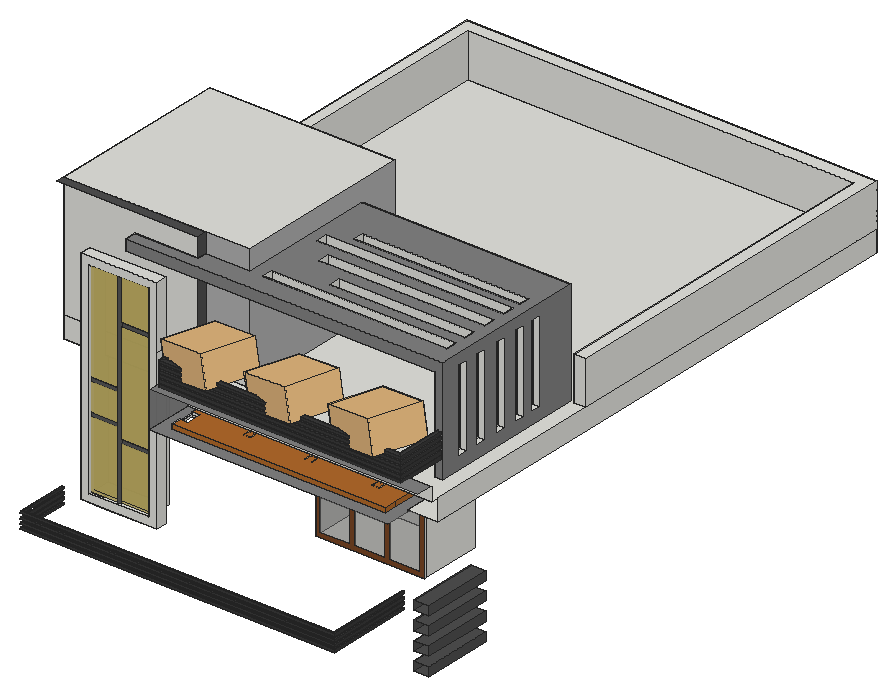
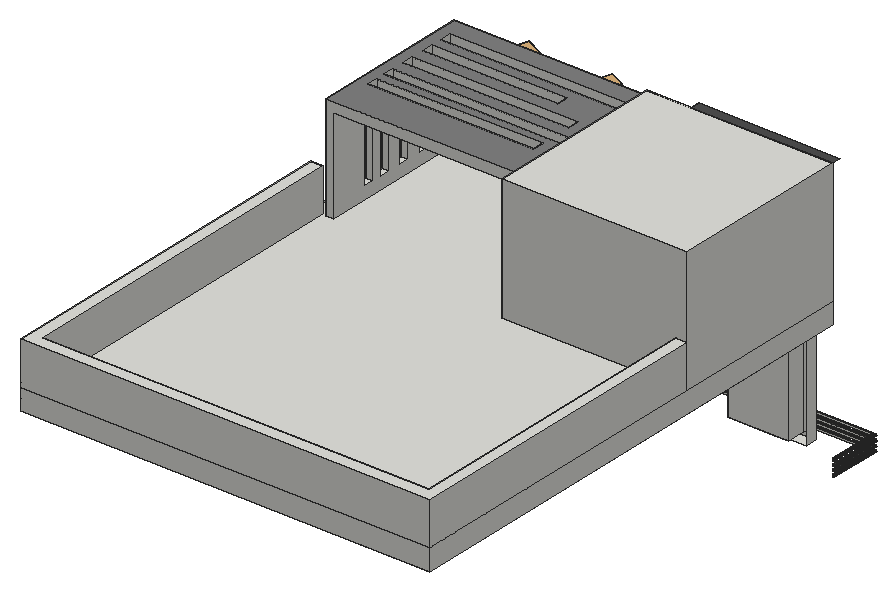
# SketchUp Ruby script. Lengths in inches.
U = 1.inch
M = Sketchup.active_model
def pt(a) = Geom::Point3d.new(a.map { |v| v * U })
def face(e, loops, mat)
  f = e.add_face(loops[0].map { |a| pt(a) })
  loops[1..].each { |l| e.add_face(l.map { |a| pt(a) }).erase! }
  f.material = f.back_material = mat if mat
  f
end
# faces: each face lists its corners as indices into pts; further lists are holes
def faces(e, pts, list, mat = nil) = list.each { |f| face(e, (f[0].is_a?(Array) ? f : [f]).map { |l| l.map { |i| pts[i] } }, mat) }
# xy, xz, yz: faces in a plane at the given z, y or x. An outline is a flat list of corners, or four numbers for a rectangle; further outlines are holes
def ring(l) = l.size == 4 ? [[l[0], l[1]], [l[2], l[1]], [l[2], l[3]], [l[0], l[3]]] : l.each_slice(2).to_a
def flat(e, list, mat, &to3) = list.each { |f| face(e, (f[0].is_a?(Array) ? f : [f]).map { |l| ring(l).map { |u, v| to3.(u, v) } }, mat) }
def xy(e, z, list, mat = nil) = flat(e, list, mat) { |x, y| [x, y, z] }
def xz(e, y, list, mat = nil) = flat(e, list, mat) { |x, z| [x, y, z] }
def yz(e, x, list, mat = nil) = flat(e, list, mat) { |y, z| [x, y, z] }
def lines(e, pts, list) = list.each { |a, b| e.add_line(pt(pts[a]), pt(pts[b])) }
# prism: a flat outline (further loops are holes) pulled along v
def prism(e, loops, v, mat = nil)
  f = face(e, loops, mat); d = Geom::Vector3d.new(v.map { |x| x * U })
  f.pushpull(f.normal.samedirection?(d) ? d.length : -d.length)
end
def box(e, o, s, mat = nil) = prism(e, [[o, [o[0] + s[0], o[1], o[2]], [o[0] + s[0], o[1] + s[1], o[2]], [o[0], o[1] + s[1], o[2]]]], [0, 0, s[2]], mat)
def at(x, y, z, deg = 0) = Geom::Transformation.translation(pt([x, y, z])) * Geom::Transformation.rotation(ORIGIN, Z_AXIS, deg.degrees)
def axes(o, x, y, z) = Geom::Transformation.new([*x, 0, *y, 0, *z, 0, *pt(o).to_a, 1])
def part(name) = M.definitions.add(name)
# library, detail: a bought-in or finely detailed component or shape, given as its bounding box
def library(name, o, s) = part(name).tap { |d| box(d.entities, o, s) }
def detail(e, o, s) = box(e.add_group.entities, o, s)
def put(e, d, t, mat = nil) = e.add_instance(d, t).tap { |i| i.material = mat if mat }
def group(e, t, mat = nil) = e.add_group.tap { |g| g.transformation = t; g.material = mat if mat }.entities
root = M.entities
M.materials.add("Generic").color = [129, 129, 129]
M.materials["Generic"].alpha = 0.97
M.materials.add("Generic\#1").color = [79, 79, 79]
M.materials.add("Generic\#4").color = [176, 176, 176]
M.materials.add("Generic\#6").color = [129, 129, 129]
M.materials.add("Material__1").color = [190, 136, 85]
M.materials.add("Material__2").color = [51, 42, 44]
M.materials.add("Material__3").color = [119, 136, 107]
M.materials.add("[Color M06]").color = [86, 86, 86]
M.materials.add("[Color M07]").color = [196, 178, 100]
M.materials["[Color M07]"].alpha = 0.86
M.materials.add("[Color M07]1").color = [58, 58, 58]
M.materials.add("[Translucent Glass Gray]").color = [128, 128, 128]
M.materials["[Translucent Glass Gray]"].alpha = 0.28
M.materials.add("[Wood Bamboo]").color = [177, 105, 43]
M.materials.add("[Wood Veneer 01]").color = [120, 70, 37]
c1 = library("Tlon Light 450 Ceiling 152 006",[-8.86,-8.86,-3.78],[17.72,17.72,3.56])
c2 = library("\#2",[-119.83,-119.83,113.8],[239.66,239.66,17.4])
c3 = library("\#4",[-204.92,-212.35,-236.71],[424.28,257.5,472.53])
c4 = part("\#3")
put(c4.entities,c3,axes([-0.37,309.72,0],[1.36765,0,0],[0,1.36765,0],[0,0,1.36765]),"Material__3")
c5 = library("\#1",[-174.07,-174.07,0],[348.14,348.14,140])
c6 = part("9")
put(c6.entities,c2,at(-19.94,-24.66,0),"Material__2")
put(c6.entities,c4,axes([17.67,-32.6,40.29],[0.29694,0.9549,0],[-0.21403,0.06656,0.97456],[0.9306,-0.28939,0.22414]))
put(c6.entities,c5,at(-19.94,-24.66,0),"Material__1")
xy(root,181.49,[[80.31,70.4,80.31,115.77,82.18,115.77,82.18,72.28,354.41,72.28,354.41,146.83,356.29,146.83,356.29,70.4]])
xy(root,181.63,[[415.03,84.21,427.87,146.83]],"Generic\#1")
xy(root,183.35,[[80.32,70.42,356.27,70.42,356.27,146.83,354.4,146.83,354.4,72.29,82.2,72.29,82.2,115.77,80.32,115.77]],"[Color M07]1")
xy(root,185.61,[[80.31,70.4,80.31,115.77,82.18,115.77,82.18,72.28,354.41,72.28,354.41,146.83,356.29,146.83,356.29,70.4]])
xy(root,187.48,[[80.32,70.42,356.27,70.42,356.27,146.83,354.4,146.83,354.4,72.29,82.2,72.29,82.2,115.77,80.32,115.77]],"[Color M07]1")
xy(root,189.57,[[415.03,84.21,427.87,146.83]],"Generic\#1")
xy(root,189.67,[[80.31,70.4,80.31,115.77,82.18,115.77,82.18,72.28,354.41,72.28,354.41,146.83,356.29,146.83,356.29,70.4]])
xy(root,191.54,[[80.32,70.42,356.27,70.42,356.27,146.83,354.4,146.83,354.4,72.29,82.2,72.29,82.2,115.77,80.32,115.77]],"[Color M07]1")
xy(root,194.11,[[80.31,70.4,80.31,115.77,82.18,115.77,82.18,72.28,354.41,72.28,354.41,146.83,356.29,146.83,356.29,70.4]])
xy(root,195.98,[[80.32,70.42,356.27,70.42,356.27,146.83,354.4,146.83,354.4,72.29,82.2,72.29,82.2,115.77,80.32,115.77]],"[Color M07]1")
xy(root,197.51,[[415.03,84.21,427.87,146.83]],"Generic\#1")
xy(root,197.89,[[104.69,106.33,123.1,115.77],[123.1,106.33,171.4,115.77]])
xy(root,204.75,[[111.55,106.33,123.1,127.83],[123.1,106.33,164.55,127.83]])
xy(root,205.44,[[415.03,84.21,427.87,146.83]],"Generic\#1")
xy(root,213.38,[[415.03,84.21,427.87,146.83]],"Generic\#1")
xy(root,214.58,[[280.99,146.83,376.49,199.39]])
xy(root,221.32,[[415.03,84.21,427.87,146.83]],"Generic\#1")
xy(root,229.26,[[415.03,84.21,427.87,146.83]],"Generic\#1")
xy(root,237.19,[[415.03,84.21,427.87,146.83]],"Generic\#1")
xy(root,258.79,[[273.73,152.11,299.55,184.17]])
xy(root,271.54,[[171.75,194.96,221.4375,227.77]])
xy(root,297.7,[[280.99,146.83,376.49,199.39]])
xy(root,304.8125,[[[200.23,62.71,200.23,194.96,273.73,194.96,273.73,146.83,409.3,146.83,409.3,62.71],[210.94,73.41,398.59,73.41,398.59,136.125,210.94,136.125,210.94,95.44,209.8,95.44,209.8,81.79,210.94,81.79]]],"Generic\#6")
xy(root,306.4375,[[209.8,81.79,210.94,95.44],[409.3,84.21,435.86,146.83],[75.86,124.21,200.23,194.96],[273.73,146.83,273.73,194.96,75.86,194.96,75.86,565.96,435.86,565.96,435.86,146.83]])
xy(root,308.875,[[210.94,73.41,210.94,81.79,218.24,81.79,218.24,95.44,210.94,95.44,210.94,136.125,398.59,136.125,398.59,73.41]],"[Wood Bamboo]")
xy(root,324.875,[[[221.17,77.89,435.86,77.89,435.86,246.92,425.3,246.92,425.3,554.58,86.17,554.58,86.17,283.64,239.11,283.64,239.11,124.21,221.17,124.21],[416.05,106.33,422.42,246.92]],[75.86,124.21,239.11,283.64],[425.3,246.92,425.3,554.58,86.17,554.58,86.17,283.64,75.86,283.64,75.86,565.96,435.86,565.96,435.86,246.92]])
xy(root,335.41,[[416.05,123.64,422.42,133.52],[416.05,143.27,422.42,153.14],[416.05,164.89,422.42,174.77],[416.05,185.71,422.42,195.58],[416.05,203.33,422.42,213.21]])
xy(root,336.625,[[200.23,62.71,435.86,62.71,435.86,77.89,221.17,77.89,221.17,124.21,200.23,124.21]],"Generic")
xy(root,342.02,[[209.05,61.9375,209.05,124.21,212.55,124.21,212.55,65.4375]])
xy(root,344.58,[[209.05,61.92,212.55,65.42,212.55,124.21,209.05,124.21]],"[Color M07]1")
xy(root,345.83,[[208.8,61.9375,208.8,124.21,212.3,124.21,212.3,65.4375]])
xy(root,348.39,[[208.8,61.92,212.3,65.42,212.3,124.21,208.8,124.21]],"[Color M07]1")
xy(root,349.96,[[208.86,61.94,208.86,124.21,212.36,124.21,212.36,65.44]])
xy(root,352.52,[[208.86,61.92,212.36,65.42,212.36,124.21,208.86,124.21]],"[Color M07]1")
xy(root,353.46,[[209.05,61.94,209.05,124.21,212.55,124.21,212.55,65.44]])
xy(root,356.02,[[209.05,61.92,212.55,65.42,212.55,124.21,209.05,124.21]],"[Color M07]1")
xy(root,357.08,[[209.05,61.94,209.05,124.21,212.55,124.21,212.55,65.44]])
xy(root,359.64,[[209.05,61.92,212.55,65.42,212.55,124.21,209.05,124.21]],"[Color M07]1")
xy(root,361.39,[[209.05,61.9375,209.05,124.21,212.55,124.21,212.55,65.4375]])
xy(root,362.9375,[[425.3,246.92,435.86,246.92,435.86,565.96,75.86,565.96,75.86,283.64,86.17,283.64,86.17,554.58,425.3,554.58]])
xy(root,363.96,[[209.05,61.92,212.55,65.42,212.55,124.21,209.05,124.21]],"[Color M07]1")
xy(root,385.04,[[111.55,106.33,164.55,127.83]])
xy(root,391.89,[[104.69,106.33,171.4,115.77]])
xy(root,407.6,[[416.05,123.64,422.42,133.52],[416.05,143.27,422.42,153.14],[416.05,164.89,422.42,174.77],[416.05,185.71,422.42,195.58],[416.05,203.33,422.42,213.21]])
xy(root,407.6,[[[144.48,106.33,144.48,115.77,200.23,115.77,200.23,124.21,239.11,124.21,239.11,246.92,416.05,246.92,416.05,106.33],[248.49,185.71,412.51,195.58],[251.05,123.64,412.51,133.52],[267.3,203.33,412.51,213.21],[267.3,164.89,412.51,174.77],[293.99,143.27,412.51,153.14]]],"Generic")
xy(root,417.1,[[[144.48,106.33,422.42,106.33,422.42,246.92,239.11,246.92,239.11,124.21,200.23,124.21,200.23,115.77,144.48,115.77],[248.49,185.71,412.51,195.58],[251.05,123.64,412.51,133.52],[267.3,203.33,412.51,213.21],[267.3,164.89,412.51,174.77],[293.99,143.27,412.51,153.14]]],"Generic\#6")
xy(root,434,[[75.86,124.21,239.11,283.64]])
xy(root,434,[[75.86,115.77,200.23,124.21]],"Generic\#1")
xz(root,73.41,[[210.94,304.8125,398.59,308.875]],"[Wood Bamboo]")
xz(root,77.89,[[221.17,324.875,435.86,336.625]])
xz(root,81.79,[[209.8,304.8125,210.94,306.4375]])
xz(root,95.44,[[209.8,304.8125,210.94,306.4375],[210.94,304.8125,218.24,306.4375],[210.94,306.4375,218.24,308.875]])
xz(root,106.33,[[[104.69,197.89,171.4,391.89],[111.55,204.75,164.55,385.04]]])
xz(root,106.33,[[[416.05,324.875,422.42,324.875,422.42,417.1,144.48,417.1,144.48,407.6,416.05,407.6],[421.36,355.49,417.86,355.54,417.9,358.1,421.4,358.05],[421.36,351.86,417.86,351.92,417.9,354.48,421.4,354.43],[421.37,340.43,417.87,340.48,417.91,343.04,421.41,342.99],[421.17,348.36,417.68,348.42,417.71,350.98,421.21,350.93],[421.37,359.8,417.87,359.85,417.91,362.42,421.41,362.36],[421.12,344.23,417.62,344.29,417.66,346.85,421.16,346.8]]],"Generic\#6")
xz(root,115.77,[[80.31,181.49,80.32,183.35,82.2,183.35,82.18,181.49],[80.31,185.61,80.32,187.48,82.2,187.48,82.18,185.61],[80.31,189.67,80.32,191.54,82.2,191.54,82.18,189.67],[80.31,194.11,80.32,195.98,82.2,195.98,82.18,194.11],[144.48,407.6,200.23,417.1]])
xz(root,123.64,[[416.05,335.41,422.42,407.6],[251.05,407.6,412.51,417.1]])
xz(root,124.21,[[75.86,306.4375,200.23,324.875],[75.86,324.875,200.23,434],[200.23,324.875,221.17,336.625],[221.17,324.875,239.11,336.625],[209.05,342.02,212.55,344.58],
  [208.8,345.83,212.3,348.39],[208.86,349.96,212.36,352.52],[209.05,353.46,212.55,356.02],[209.05,357.08,212.55,359.64],[209.05,361.39,212.55,363.96]])
xz(root,124.21,[[[200.23,336.625,239.11,407.6],[209.05,357.08,212.55,359.64],[209.05,353.46,212.55,356.02],[208.86,349.96,212.36,352.52],[208.8,345.83,212.3,348.39],[209.05,342.02,212.55,344.58],[209.05,361.39,212.55,363.96]],[200.23,417.1,239.11,434]],"Generic\#4")
xz(root,127.83,[[111.55,204.75,164.55,385.04]])
xz(root,133.52,[[416.05,335.41,422.42,407.6],[251.05,407.6,412.51,417.1]])
xz(root,136.125,[[210.94,304.8125,398.59,308.875]],"[Wood Bamboo]")
xz(root,143.27,[[416.05,335.41,422.42,407.6],[293.99,407.6,412.51,417.1]])
xz(root,146.83,[[273.73,304.8125,409.3,306.4375]])
xz(root,153.14,[[416.05,335.41,422.42,407.6],[293.99,407.6,412.51,417.1]])
xz(root,164.89,[[416.05,335.41,422.42,407.6],[267.3,407.6,412.51,417.1]])
xz(root,174.77,[[416.05,335.41,422.42,407.6],[267.3,407.6,412.51,417.1]])
xz(root,185.71,[[416.05,335.41,422.42,407.6],[248.49,407.6,412.51,417.1]])
xz(root,194.96,[[200.23,304.8125,273.73,306.4375]])
xz(root,195.58,[[416.05,335.41,422.42,407.6],[248.49,407.6,412.51,417.1]])
xz(root,199.39,[[280.99,214.58,376.49,297.7]])
xz(root,203.33,[[416.05,335.41,422.42,407.6],[267.3,407.6,412.51,417.1]])
xz(root,213.21,[[416.05,335.41,422.42,407.6],[267.3,407.6,412.51,417.1]])
xz(root,246.92,[[416.05,324.875,416.05,407.6,239.11,407.6,239.11,417.1,422.42,417.1,422.42,324.875],[425.3,324.875,435.86,362.9375]])
xz(root,283.64,[[86.17,324.875,86.17,362.9375,75.86,362.9375,75.86,434,239.11,434,239.11,324.875]])
xz(root,554.58,[[86.17,324.875,425.3,362.9375]])
xz(root,565.96,[[75.86,306.4375,435.86,324.875],[75.86,324.875,435.86,362.9375]])
yz(root,75.86,[[124.21,306.4375,565.96,324.875],[124.21,324.875,283.64,434],[283.64,324.875,565.96,362.9375]])
yz(root,86.17,[[283.64,324.875,554.58,362.9375]])
yz(root,104.69,[[106.33,197.89,115.77,391.89]])
yz(root,111.55,[[106.33,204.75,127.83,385.04]])
yz(root,144.48,[[106.33,407.6,115.77,417.1]])
yz(root,164.55,[[106.33,204.75,127.83,306.4375],[106.33,306.4375,127.83,336.625],[106.33,336.625,127.83,385.04]])
yz(root,171.4,[[106.33,197.89,115.77,306.4375],[106.33,306.4375,115.77,336.625],[106.33,336.625,115.77,391.89]])
yz(root,200.23,[[115.77,304.8125,124.21,336.625],[124.21,304.8125,194.96,306.4375],[115.77,407.6,124.21,417.1]])
yz(root,200.23,[[62.71,304.8125,115.77,336.625]],"Generic")
yz(root,200.23,[[115.77,336.625,124.21,407.6],[115.77,417.1,124.21,434]],"Generic\#1")
yz(root,208.8,[[61.9375,345.83,61.92,348.39,124.21,348.39,124.21,345.83]],"[Color M07]1")
yz(root,208.86,[[61.94,349.96,61.92,352.52,124.21,352.52,124.21,349.96]],"[Color M07]1")
yz(root,209.05,[[61.9375,342.02,61.92,344.58,124.21,344.58,124.21,342.02],[61.94,353.46,61.92,356.02,124.21,356.02,124.21,353.46],[61.94,357.08,61.92,359.64,124.21,359.64,124.21,357.08],[61.9375,361.39,61.92,363.96,124.21,363.96,124.21,361.39]],"[Color M07]1")
yz(root,209.8,[[81.79,304.8125,95.44,306.4375]])
yz(root,210.94,[[73.41,304.8125,81.79,308.875],[81.79,304.8125,95.44,306.4375]])
yz(root,210.94,[[95.44,304.8125,136.125,308.875]],"[Wood Bamboo]")
yz(root,212.3,[[65.4375,345.83,124.21,345.83,124.21,348.39,65.42,348.39]],"[Color M07]1")
yz(root,212.36,[[65.44,349.96,124.21,349.96,124.21,352.52,65.42,352.52]],"[Color M07]1")
yz(root,212.55,[[65.4375,342.02,124.21,342.02,124.21,344.58,65.42,344.58],[65.44,353.46,124.21,353.46,124.21,356.02,65.42,356.02],[65.44,357.08,124.21,357.08,124.21,359.64,65.42,359.64],[65.4375,361.39,124.21,361.39,124.21,363.96,65.42,363.96]],"[Color M07]1")
yz(root,221.17,[[77.89,324.875,124.21,336.625]])
yz(root,239.11,[[124.21,324.875,283.64,324.875,283.64,434,124.21,434,124.21,417.1,246.92,417.1,246.92,407.6,124.21,407.6]],"Generic\#4")
yz(root,248.49,[[185.71,407.6,195.58,417.1]])
yz(root,251.05,[[123.64,407.6,133.52,417.1]])
yz(root,267.3,[[164.89,407.6,174.77,417.1],[203.33,407.6,213.21,417.1]])
yz(root,273.73,[[146.83,304.8125,194.96,306.4375]])
yz(root,280.99,[[146.83,214.58,199.39,297.7]])
yz(root,293.99,[[143.27,407.6,153.14,417.1]])
yz(root,376.49,[[146.83,214.58,199.39,297.7]])
yz(root,398.59,[[73.41,304.8125,84.21,308.875],[84.21,304.8125,136.125,308.875]],"[Wood Bamboo]")
yz(root,409.3,[[84.21,304.8125,146.83,306.4375]],"Generic\#6")
yz(root,412.51,[[123.64,407.6,133.52,417.1],[143.27,407.6,153.14,417.1],[164.89,407.6,174.77,417.1],[185.71,407.6,195.58,417.1],[203.33,407.6,213.21,417.1]])
yz(root,415.03,[[84.21,181.63,146.83,189.57],[84.21,197.51,146.83,205.44],[84.21,213.38,146.83,221.32],[84.21,229.26,146.83,237.19]],"Generic\#1")
yz(root,416.05,[[106.33,324.875,106.33,407.6,123.64,407.6,123.64,335.41,133.52,335.41,133.52,407.6,143.27,407.6,143.27,335.41,153.14,335.41,153.14,407.6,164.89,407.6,164.89,335.41,174.77,335.41,174.77,407.6,185.71,407.6,185.71,335.41,195.58,335.41,195.58,407.6,203.33,407.6,203.33,335.41,213.21,335.41,213.21,407.6,246.92,407.6,246.92,324.875]])
yz(root,422.42,[[[106.33,324.875,246.92,417.1],[203.33,335.41,213.21,407.6],[164.89,335.41,174.77,407.6],[143.27,335.41,153.14,407.6],[123.64,335.41,133.52,407.6],[185.71,335.41,195.58,407.6]]],"Generic\#6")
yz(root,425.3,[[246.92,324.875,554.58,362.9375]])
yz(root,427.87,[[84.21,181.63,146.83,189.57],[84.21,197.51,146.83,205.44],[84.21,213.38,146.83,221.32],[84.21,229.26,146.83,237.19]],"Generic\#1")
yz(root,435.86,[[84.21,306.4375,565.96,324.875],[246.92,324.875,565.96,362.9375]])
p = [[80.32,115.77,183.35],[80.31,115.77,181.49],[80.31,70.4,181.49],[80.32,70.42,183.35],[356.29,70.4,181.49],[356.27,70.42,183.35],
  [356.29,146.83,181.49],[356.27,146.83,183.35],[82.18,115.77,181.49],[82.2,115.77,183.35],[82.2,72.29,183.35],[82.18,72.28,181.49],
  [354.4,72.29,183.35],[354.41,72.28,181.49],[354.4,146.83,183.35],[354.41,146.83,181.49],[80.32,115.77,187.48],[80.31,115.77,185.61],
  [80.31,70.4,185.61],[80.32,70.42,187.48],[356.29,70.4,185.61],[356.27,70.42,187.48],[356.29,146.83,185.61],[356.27,146.83,187.48],
  [82.18,115.77,185.61],[82.2,115.77,187.48],[82.2,72.29,187.48],[82.18,72.28,185.61],[354.4,72.29,187.48],[354.41,72.28,185.61],
  [354.4,146.83,187.48],[354.41,146.83,185.61],[80.32,115.77,191.54],[80.31,115.77,189.67],[80.31,70.4,189.67],[80.32,70.42,191.54],
  [356.29,70.4,189.67],[356.27,70.42,191.54],[356.29,146.83,189.67],[356.27,146.83,191.54],[82.18,115.77,189.67],[82.2,115.77,191.54],
  [82.2,72.29,191.54],[82.18,72.28,189.67],[354.4,72.29,191.54],[354.41,72.28,189.67],[354.4,146.83,191.54],[354.41,146.83,189.67],
  [80.32,115.77,195.98],[80.31,115.77,194.11],[80.31,70.4,194.11],[80.32,70.42,195.98],[356.29,70.4,194.11],[356.27,70.42,195.98],
  [356.29,146.83,194.11],[356.27,146.83,195.98],[82.18,115.77,194.11],[82.2,115.77,195.98],[82.2,72.29,195.98],[82.18,72.28,194.11],
  [354.4,72.29,195.98],[354.41,72.28,194.11],[354.4,146.83,195.98],[354.41,146.83,194.11],[209.05,61.9375,342.02],[212.55,65.4375,342.02],
  [417.87,65.4375,340.48],[421.37,61.9375,340.43],[209.05,61.92,344.58],[421.41,61.92,342.99],[417.87,106.33,340.48],[421.37,106.33,340.43],
  [421.41,106.33,342.99],[212.55,65.42,344.58],[417.91,65.42,343.04],[417.91,106.33,343.04],[208.8,61.9375,345.83],[212.3,65.4375,345.83],
  [417.62,65.4375,344.29],[421.12,61.9375,344.23],[208.8,61.92,348.39],[421.16,61.92,346.8],[417.62,106.33,344.29],[421.12,106.33,344.23],
  [421.16,106.33,346.8],[212.3,65.42,348.39],[417.66,65.42,346.85],[417.66,106.33,346.85],[208.86,61.94,349.96],[212.36,65.44,349.96],
  [417.68,65.44,348.42],[421.17,61.94,348.36],[208.86,61.92,352.52],[421.21,61.92,350.93],[417.68,106.33,348.42],[421.17,106.33,348.36],
  [421.21,106.33,350.93],[212.36,65.42,352.52],[417.71,65.42,350.98],[417.71,106.33,350.98],[209.05,61.94,353.46],[212.55,65.44,353.46],
  [417.86,65.44,351.92],[421.36,61.94,351.86],[209.05,61.92,356.02],[421.4,61.92,354.43],[417.86,106.33,351.92],[421.36,106.33,351.86],
  [421.4,106.33,354.43],[212.55,65.42,356.02],[417.9,65.42,354.48],[417.9,106.33,354.48],[209.05,61.94,357.08],[212.55,65.44,357.08],
  [417.86,65.44,355.54],[421.36,61.94,355.49],[209.05,61.92,359.64],[421.4,61.92,358.05],[417.86,106.33,355.54],[421.36,106.33,355.49],
  [421.4,106.33,358.05],[212.55,65.42,359.64],[417.9,65.42,358.1],[417.9,106.33,358.1],[209.05,61.9375,361.39],[212.55,65.4375,361.39],
  [417.87,65.4375,359.85],[421.37,61.9375,359.8],[209.05,61.92,363.96],[421.41,61.92,362.36],[417.87,106.33,359.85],[421.37,106.33,359.8],
  [421.41,106.33,362.36],[212.55,65.42,363.96],[417.91,65.42,362.42],[417.91,106.33,362.42],[355.49,71.21,182.28],[355.49,146.83,182.28],
  [81.11,71.21,182.28],[81.11,115.77,182.28],[355.49,71.21,186.47],[355.49,146.83,186.47],[81.11,71.21,186.47],[81.11,115.77,186.47],
  [355.49,71.21,190.65],[355.49,146.83,190.65],[81.11,71.21,190.65],[81.11,115.77,190.65],[355.49,71.21,194.84],[355.49,146.83,194.84],
  [81.11,71.21,194.84],[81.11,115.77,194.84],[412.51,213.21,407.6],[416.05,213.21,407.6],[412.51,195.58,407.6],[416.05,195.58,407.6],
  [412.51,174.77,407.6],[416.05,174.77,407.6],[412.51,153.14,407.6],[416.05,153.14,407.6],[412.51,133.52,407.6],[416.05,133.52,407.6],
  [210.39,124.21,343.01],[210.39,63.27,343.01],[420.05,106.33,341.43],[420.05,63.27,341.43],[210.14,124.21,346.8125],[210.14,63.27,346.8125],
  [419.8,106.33,345.24],[419.8,63.27,345.24],[210.2,124.21,351.38],[210.2,63.27,351.38],[419.86,106.33,349.81],[419.86,63.27,349.81],
  [210.39,124.21,355.07],[210.39,63.27,355.07],[420.05,106.33,353.5],[420.05,63.27,353.5],[210.39,124.21,358.76],[210.39,63.27,358.76],
  [420.05,106.33,357.18],[420.05,63.27,357.18],[210.39,124.21,362.44],[210.39,63.27,362.44],[420.05,106.33,360.87],[420.05,63.27,360.87]]
faces(root,p,[[0,1,2,3],[3,2,4,5],[5,4,6,7],[8,9,10,11],[13,12,14,15],[16,17,18,19],[19,18,20,21],[21,20,22,23],
  [24,25,26,27],[29,28,30,31],[32,33,34,35],[35,34,36,37],[37,36,38,39],[40,41,42,43],[45,44,46,47],[48,49,50,51],
  [51,50,52,53],[53,52,54,55],[56,57,58,59],[61,60,62,63],[68,64,67,69],[69,67,71,72],[66,74,75,70],[73,68,69,74],
  [74,69,72,75],[80,76,79,81],[81,79,83,84],[78,86,87,82],[85,80,81,86],[86,81,84,87],[92,88,91,93],[93,91,95,96],
  [90,98,99,94],[97,92,93,98],[98,93,96,99],[104,100,103,105],[105,103,107,108],[102,110,111,106],[109,104,105,110],[110,105,108,111],
  [116,112,115,117],[117,115,119,120],[114,122,123,118],[121,116,117,122],[122,117,120,123],[128,124,127,129],[129,127,131,132],[126,134,135,130],
  [133,128,129,134],[134,129,132,135]],"[Color M07]1")
faces(root,p,[[11,10,12,13],[27,26,28,29],[43,42,44,45],[59,58,60,61],[64,65,66,67],[67,66,70,71],[65,73,74,66],[76,77,78,79],
  [79,78,82,83],[77,85,86,78],[88,89,90,91],[91,90,94,95],[89,97,98,90],[100,101,102,103],[103,102,106,107],[101,109,110,102],
  [112,113,114,115],[115,114,118,119],[113,121,122,114],[124,125,126,127],[127,126,130,131],[125,133,134,126]])
lines(root,p,[[136,137],[138,136],[139,138],[140,141],[142,140],[143,142],[144,145],[146,144],[147,146],[148,149],[150,148],[151,150],
  [152,153],[154,155],[156,157],[158,159],[160,161],[162,163],[164,165],[165,163],[166,167],[168,169],[169,167],[170,171],
  [172,173],[173,171],[174,175],[176,177],[177,175],[178,179],[180,181],[181,179],[182,183],[184,185],[185,183]])
g1 = group(root,at(110.45,108.83,204.75))
xy(g1,0,[[0,0,11.55,3],[11.55,0,53,3]])
xy(g1,180.29,[[0,0,53,3]])
xz(g1,0,[[25,0,28,180.29],[28,47.84,53,50.84],[0,59.75,25,62.75],[0,87.56,25,90.56],[28,139.72,53,142.72]],"[Color M06]")
xz(g1,0,[[0,0,25,59.75],[28,0,53,47.84],[28,50.84,53,139.72],[0,62.75,25,87.56],[0,90.56,25,180.29],
  [28,142.72,53,180.29]],"[Color M07]")
xz(g1,3,[[0,0,53,180.29]],"[Color M07]")
yz(g1,0,[[0,0,3,180.29]])
yz(g1,53,[[0,0,3,101.6875],[0,101.6875,3,131.875],[0,131.875,3,180.29]])
g2 = group(root,at(280.99,143.83,214.58))
xy(g2,0,[[0,0,95.5,3]])
xy(g2,83.125,[[0,0,95.5,3]])
xz(g2,0,[[4.0625,4.0625,30.48,79.0625],[34.54,4.0625,60.96,79.0625],[65.02,4.0625,91.4375,79.0625]],"[Translucent Glass Gray]")
xz(g2,0,[[[0,0,95.5,83.125],[65.02,4.0625,91.4375,79.0625],[34.54,4.0625,60.96,79.0625],[4.0625,4.0625,30.48,79.0625]]],"[Wood Veneer 01]")
xz(g2,3,[[0,0,95.5,83.125]],"[Translucent Glass Gray]")
yz(g2,0,[[0,0,3,83.125]])
yz(g2,95.5,[[0,0,3,83.125]])
put(root,c1,axes([315.84,95.73,308.95],[0.35,0,0],[0,0.35,0],[0,0,0.35]))
put(root,c1,axes([374.65,95.73,308.95],[0.35,0,0],[0,0.35,0],[0,0,0.35]))
put(root,c1,axes([261.59,95.73,308.95],[0.35,0,0],[0,0.35,0],[0,0,0.35]))
put(root,c6,axes([238.98,83.66,349.59],[0.078,0,0],[0,0.078,0],[0,0,0.078]))
put(root,c6,axes([312.67,83.66,349.59],[0.078,0,0],[0,0.078,0],[0,0,0.078]))
put(root,c6,axes([385.92,83.66,349.59],[0.078,0,0],[0,0.078,0],[0,0,0.078]))
put(root,c1,axes([288.89,159.06,407.92],[0.35,0,0],[0,0.35,0],[0,0,0.35]))
put(root,c1,axes([331.57,159.06,407.92],[0.35,0,0],[0,0.35,0],[0,0,0.35]))
put(root,c1,axes([374.26,159.06,407.92],[0.35,0,0],[0,0.35,0],[0,0,0.35]))
put(root,c1,axes([331.57,114.49,407.92],[0.35,0,0],[0,0.35,0],[0,0,0.35]))
put(root,c1,axes([288.89,114.49,407.92],[0.35,0,0],[0,0.35,0],[0,0,0.35]))
put(root,c1,axes([374.26,114.49,407.92],[0.35,0,0],[0,0.35,0],[0,0,0.35]))
